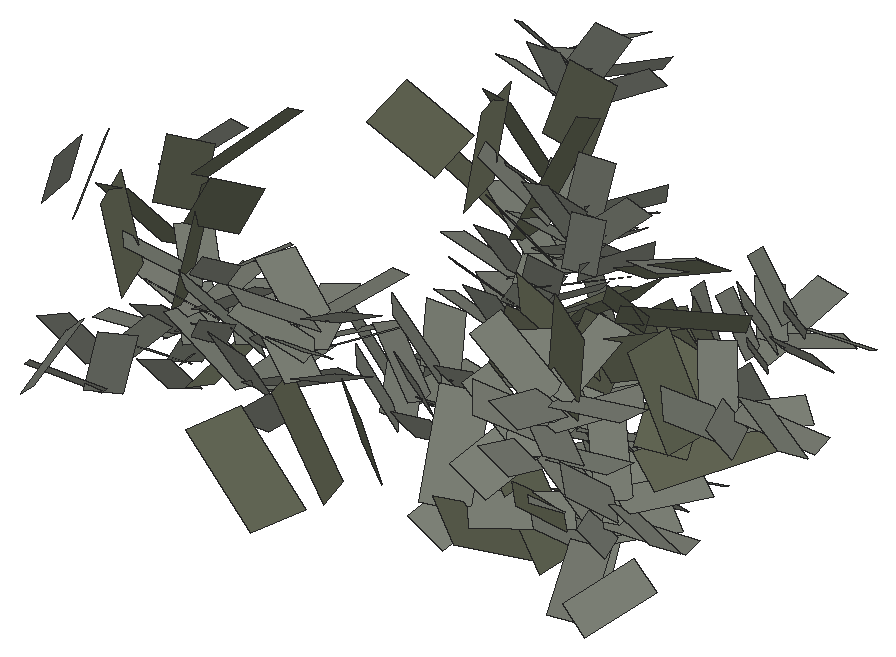
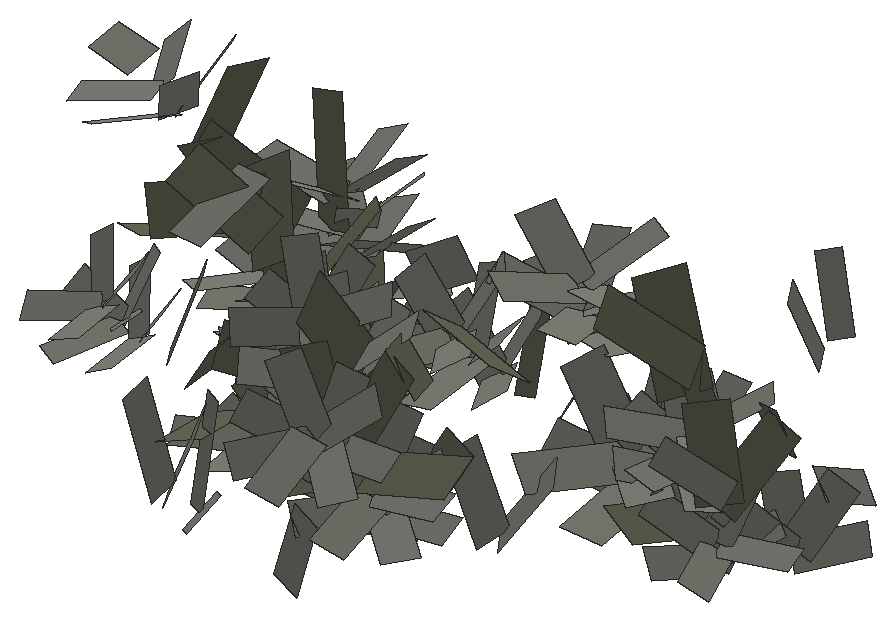
# SketchUp Ruby script. Lengths in inches.
U = 1.inch
M = Sketchup.active_model
def pt(a) = Geom::Point3d.new(a.map { |v| v * U })
def face(e, loops, mat)
  f = e.add_face(loops[0].map { |a| pt(a) })
  loops[1..].each { |l| e.add_face(l.map { |a| pt(a) }).erase! }
  f.material = f.back_material = mat if mat
  f
end
# faces: each face lists its corners as indices into pts; further lists are holes
def faces(e, pts, list, mat = nil) = list.each { |f| face(e, (f[0].is_a?(Array) ? f : [f]).map { |l| l.map { |i| pts[i] } }, mat) }
# xy, xz, yz: faces in a plane at the given z, y or x. An outline is a flat list of corners, or four numbers for a rectangle; further outlines are holes
def ring(l) = l.size == 4 ? [[l[0], l[1]], [l[2], l[1]], [l[2], l[3]], [l[0], l[3]]] : l.each_slice(2).to_a
def flat(e, list, mat, &to3) = list.each { |f| face(e, (f[0].is_a?(Array) ? f : [f]).map { |l| ring(l).map { |u, v| to3.(u, v) } }, mat) }
def xy(e, z, list, mat = nil) = flat(e, list, mat) { |x, y| [x, y, z] }
def xz(e, y, list, mat = nil) = flat(e, list, mat) { |x, z| [x, y, z] }
def yz(e, x, list, mat = nil) = flat(e, list, mat) { |y, z| [x, y, z] }
def lines(e, pts, list) = list.each { |a, b| e.add_line(pt(pts[a]), pt(pts[b])) }
# prism: a flat outline (further loops are holes) pulled along v
def prism(e, loops, v, mat = nil)
  f = face(e, loops, mat); d = Geom::Vector3d.new(v.map { |x| x * U })
  f.pushpull(f.normal.samedirection?(d) ? d.length : -d.length)
end
def box(e, o, s, mat = nil) = prism(e, [[o, [o[0] + s[0], o[1], o[2]], [o[0] + s[0], o[1] + s[1], o[2]], [o[0], o[1] + s[1], o[2]]]], [0, 0, s[2]], mat)
def at(x, y, z, deg = 0) = Geom::Transformation.translation(pt([x, y, z])) * Geom::Transformation.rotation(ORIGIN, Z_AXIS, deg.degrees)
def axes(o, x, y, z) = Geom::Transformation.new([*x, 0, *y, 0, *z, 0, *pt(o).to_a, 1])
def part(name) = M.definitions.add(name)
# library, detail: a bought-in or finely detailed component or shape, given as its bounding box
def library(name, o, s) = part(name).tap { |d| box(d.entities, o, s) }
def detail(e, o, s) = box(e.add_group.entities, o, s)
def put(e, d, t, mat = nil) = e.add_instance(d, t).tap { |i| i.material = mat if mat }
def group(e, t, mat = nil) = e.add_group.tap { |g| g.transformation = t; g.material = mat if mat }.entities
root = M.entities
M.materials.add("viburnumblaasdfas0df1w06d").color = [98, 102, 84]
M.materials.add("viburnumbladsadfasdfad0w122").color = [125, 129, 119]
c1 = part("Component\#314")
p = [[0.14,0,0],[2.58,0.05,0.25],[2.44,5.11,2.64],[0,5.05,2.39]]
faces(c1.entities,p,[[0,1,2,3]],"viburnumblaasdfas0df1w06d")
c2 = part("viburnumblad1\#2")
put(c2.entities,c1,axes([-37.25,6.23,19.31],[75.98784,0,0],[0,65.50676,0],[0,0,75.98784]))
c3 = part("Component\#315")
p = [[0.25,0,0],[2.05,0.01,0.35],[1.81,4.2,1.66],[0,4.19,1.3125]]
faces(c3.entities,p,[[0,1,2,3]],"viburnumbladsadfasdfad0w122")
c4 = part("viburnumblad2")
put(c4.entities,c3,axes([-19.23,-4.49,-32.18],[83.35428,0,0],[0,79.38502,0],[0,0,83.35428]))
put(root,c2,axes([2216.9,347.35,29.54],[-0.011,0.0051,0.00655],[-0.00551,-0.01483,0.0023],[0.00681,-0.00067,0.01196]))
put(root,c4,axes([2205.93,347.0625,36.3125],[-0.01209,-0.0034,-0.0003],[0.00332,-0.01209,0.00349],[-0.00129,0.00365,0.01095]))
put(root,c4,axes([2205.76,346.42,37.9],[-0.01088,0.00599,-0.0016],[-0.00628,-0.01045,0.00254],[-0.00013,0.00352,0.01104]))
put(root,c4,axes([2219.11,347.34,37.76],[-0.01207,0.00042,0.00346],[-0.00034,-0.01255,0.00035],[0.00347,0.00024,0.01207]))
put(root,c2,axes([2204.65,343.45,27.99],[0.00623,0.01349,0.00121],[-0.0157,0.00724,0.00014],[-0.00044,-0.00098,0.01352]))
put(root,c4,axes([2190.32,344.05,30.32],[0.00946,-0.00383,0.00571],[0.00246,0.01108,0.00318],[-0.00637,-0.00125,0.00808]))
put(root,c4,axes([2190.61,347.02,39.96],[0.00021,-0.01046,-0.0046],[0.00792,-0.00325,0.00774],[-0.00831,-0.0033,0.00712]))
put(root,c4,axes([2214.1,343.22,33.47],[0.00902,0.01086,-0.00673],[-0.00719,0.01113,0.00831],[0.01056,-0.0017,0.01141]))
put(root,c4,axes([2218.1,347.48,34.8125],[-0.0126,0.00044,0.00361],[-0.00031,-0.0113,0.00032],[0.00347,0.00024,0.01207]))
put(root,c4,axes([2205.46,347.33,34.83],[-0.00597,-0.01037,0.00113],[0.01154,-0.00613,0.0032],[-0.00222,0.00293,0.01099]))
put(root,c2,axes([2207.0625,345,29.67],[-0.00512,0.01258,-0.00225],[-0.01225,-0.00318,0.00944],[0.00707,0.00483,0.00942]))
put(root,c2,axes([2217.31,348.43,31.83],[-0.01089,-0.0066,0.00527],[0.00777,-0.0139,-0.00135],[0.00514,0.00164,0.01268]))
put(root,c4,axes([2221.26,344.42,30.01],[0.00733,0.00034,-0.00907],[0.00348,0.00978,0.00299],[0.00808,-0.00497,0.00546]))
put(root,c4,axes([2220.3,344.48,29.09],[0.00746,0.0085,-0.0048],[-0.00195,0.00645,0.00799],[0.00881,-0.00455,0.00477]))
put(root,c4,axes([2214.24,344.98,33.36],[0.00842,-0.01125,-0.00685],[0.01063,0.01127,-0.00543],[0.00843,-0.00165,0.01307]))
put(root,c2,axes([2208.35,346.97,30.46],[-0.01166,0.00571,0.00452],[-0.00151,-0.01177,0.01017],[0.0071,0.00732,0.00793]))
put(root,c4,axes([2205.3,345.74,36.45],[-0.0033,0.01188,-0.00196],[-0.01112,-0.00285,0.00099],[0.00058,0.00262,0.01122]))
put(root,c4,axes([2218.33,346.89,36.22],[-0.008,0.00913,0.00324],[-0.00789,-0.00792,0.00285],[0.00448,-0.00024,0.01173]))
put(root,c4,axes([2218.32,348.36,36.4],[-0.00907,-0.00853,0.00165],[0.00877,-0.00968,-0.00184],[0.0024,-0.00017,0.01233]))
put(root,c4,axes([2205.61,347.97,37.66],[-0.00622,-0.0108,0.00117],[0.01069,-0.00568,0.00296],[-0.00222,0.00293,0.01099]))
put(root,c4,axes([2228.56,348.54,39.8],[-0.00908,-0.00254,0.00688],[0.00302,-0.01141,-0.00024],[0.00679,0.00165,0.00837]))
put(root,c4,axes([2221.14,348.53,31.72],[-0.00974,-0.00261,0.006],[0.00353,-0.01123,0.00072],[0.00551,0.00254,0.00899]))
put(root,c4,axes([2220.21,347.85,30.78],[-0.00853,0.00601,0.00433],[-0.00446,-0.01051,0.00545],[0.00645,0.00235,0.00846]))
put(root,c4,axes([2212.86,344.05,32],[0.01184,-0.00027,-0.00922],[0.00172,0.01671,0.00172],[0.00948,-0.00223,0.01224]))
put(root,c4,axes([2227.48,347.97,38.95],[-0.00764,0.00611,0.00552],[-0.0043,-0.01063,0.00535],[0.00765,0.00146,0.00773]))
put(root,c4,axes([2221.76,347.79,33.03],[-0.00889,0.00626,0.00451],[-0.00413,-0.00973,0.00504],[0.00645,0.00235,0.00846]))
put(root,c4,axes([2215.02,344.33,35.29],[0.01234,-0.00028,-0.00961],[0.00159,0.01547,0.00159],[0.00948,-0.00223,0.01224]))
put(root,c4,axes([2217.81,346.48,38.03],[0.00076,0.01249,0.00112],[-0.01157,0.00026,0.0049],[0.00485,-0.00133,0.01151]))
put(root,c4,axes([2204.4,345.6,35.14],[0.00564,0.00974,-0.00221],[-0.01091,0.00622,-0.00021],[0.00111,0.00263,0.01119]))
put(root,c4,axes([2192.31,347.93,29.6],[-0.00614,0.00518,-0.0082],[-0.00794,-0.00715,0.00088],[-0.00475,0.00709,0.00648]))
put(root,c4,axes([2190.82,347.36,38.47],[0.00662,-0.00815,0.00069],[0.00514,0.00494,0.00894],[-0.00725,-0.00529,0.00709]))
put(root,c4,axes([2217.05,346.68,35.125],[0.00022,0.01156,-0.00012],[-0.01157,0.00026,0.0049],[0.0049,0.00003,0.01157]))
put(root,c4,axes([2229.24,349.17,41],[-0.00489,-0.00995,0.00397],[0.00876,-0.00628,-0.0047],[0.00608,0.00102,0.00892]))
put(root,c2,axes([2217.91,347.02,29.08],[0.00107,0.01287,0.00071],[-0.01171,0.00034,0.00907],[0.0079,-0.00141,0.00892]))
put(root,c4,axes([2221.62,349.27,32.95],[-0.00489,-0.00995,0.00397],[0.00954,-0.00607,-0.00338],[0.00477,0.0019,0.00949]))
put(root,c4,axes([2218.31,348.66,38.125],[-0.00076,-0.01249,-0.00112],[0.01239,-0.00058,-0.00197],[0.0019,-0.00123,0.01236]))
put(root,c4,axes([2204.76,347.85,36.15],[0.0033,-0.01188,0.00196],[0.01189,0.00365,0.00167],[-0.00236,0.00179,0.01115]))
put(root,c4,axes([2217.17,348.73,35.17],[-0.00073,-0.01199,-0.00108],[0.01339,-0.00063,-0.00213],[0.0019,-0.00123,0.01236]))
put(root,c4,axes([2220.49,347.47,32.1875],[-0.00283,0.01146,0.00038],[-0.0094,-0.00257,0.00741],[0.00704,0.00146,0.00821]))
put(root,c2,axes([2224.92,347.37,37.5],[0.00184,0.01273,0.00122],[-0.0105,0.00029,0.01027],[0.00896,-0.0024,0.00784]))
put(root,c4,axes([2191.86,349.27,30.3],[-0.01,-0.00241,-0.00568],[-0.00201,-0.00892,0.00667],[-0.00557,0.00722,0.00577]))
put(root,c4,axes([2192.36,349.06,28.86],[-0.008,-0.00859,0.00017],[0.00566,-0.00462,0.00938],[-0.00647,0.00667,0.0055]))
put(root,c4,axes([2204.18,346.25,37.82],[0.00622,0.0108,-0.00117],[-0.01091,0.00622,-0.00021],[0.00044,0.00147,0.01138]))
put(root,c4,axes([2208.94,349.56,32.23],[-0.00734,-0.00647,0.00686],[0.01022,-0.00834,0.00267],[0.00284,0.00722,0.00872]))
put(root,c2,axes([2218.16,348.42,36.08],[-0.01355,0.00411,0.00465],[0.00135,-0.01078,0.01345],[0.00609,0.01091,0.00813]))
put(root,c4,axes([2208.95,348.22,33.07],[-0.00945,0.00892,-0.00145],[-0.0064,-0.00533,0.00736],[0.00487,0.007,0.00802]))
put(root,c4,axes([2200.49,349.96,31.1],[-0.01458,-0.00076,0.00047],[0.00121,-0.01217,0.00796],[0.00032,0.00837,0.01162]))
put(root,c4,axes([2209.86,349.68,33.51],[-0.01181,0.00128,0.00407],[0.00154,-0.01046,0.00743],[0.00382,0.0075,0.00815]))
put(root,c4,axes([2199.99,350.08,29.27],[-0.0086,-0.00967,0.00326],[0.01109,-0.00774,0.00569],[-0.00192,0.00675,0.01234]))
put(root,c4,axes([2219.47,346.63,29.39],[0.00909,0.00791,-0.00471],[-0.00403,0.00937,0.00796],[0.00828,-0.00412,0.00905]))
put(root,c4,axes([2196.97,350.23,33.79],[-0.01133,0.00035,-0.0015],[-0.0009,-0.01068,0.0043],[-0.00126,0.00434,0.0105]))
put(root,c4,axes([2203.76,346.59,36.26],[0.01209,0.0034,0.0003],[-0.00342,0.01218,-0.00058],[-0.00049,0.00075,0.01143]))
put(root,c4,axes([2216.64,346.95,36.74],[0.00907,0.00853,-0.00165],[-0.0076,0.009,0.00473],[0.00435,-0.00239,0.01154]))
put(root,c4,axes([2196.89,350.67,32.32],[-0.00757,-0.0073,-0.00011],[0.00727,-0.00761,0.00446],[-0.00317,0.00314,0.01053]))
put(root,c4,axes([2216.97,348.53,36.82],[0.008,-0.00913,-0.00324],[0.00942,0.00831,-0.00017],[0.00227,-0.00232,0.01214]))
put(root,c4,axes([2227.64,349.54,40.45],[0.00217,-0.01153,-0.00126],[0.00998,0.00257,-0.00587],[0.00594,-0.00007,0.00905]))
put(root,c4,axes([2204.03,347.81,37.58],[0.01088,-0.00599,0.0016],[0.00606,0.01099,0.00021],[-0.00165,0.00089,0.01133]))
put(root,c4,axes([2220.1,349.52,32.21],[0.00283,-0.01146,-0.00038],[0.01049,0.00275,-0.00491],[0.00467,0.00082,0.00968]))
put(root,c4,axes([2218.96,347.65,31.57],[0.0051,0.01038,-0.00415],[-0.00729,0.00572,0.00502],[0.00694,0.00038,0.0084]))
put(root,c4,axes([2226.33,347.78,39.87],[0.0051,0.01038,-0.00415],[-0.00633,0.00571,0.00604],[0.00802,-0.00053,0.00751]))
put(root,c4,axes([2199.9,349.96,33.125],[-0.01112,0.00864,-0.0042],[-0.00937,-0.00881,0.00635],[0.00161,0.00797,0.01181]))
put(root,c4,axes([2220.49,347.71,33.79],[0.00489,0.00995,-0.00397],[-0.0081,0.00635,0.00558],[0.00694,0.00038,0.0084]))
put(root,c4,axes([2196.19,349.92,35.3],[-0.00749,0.00804,-0.00315],[-0.00863,-0.00712,0.00235],[-0.00031,0.00392,0.01074]))
put(root,c4,axes([2210.16,349.75,35.19],[-0.00905,0.00854,-0.00139],[-0.00711,-0.00593,0.00818],[0.00487,0.007,0.00802]))
put(root,c4,axes([2210.29,351.07,34.36],[-0.00765,-0.00673,0.00714],[0.00947,-0.00772,0.00247],[0.00284,0.00722,0.00872]))
put(root,c4,axes([2217.01,347.8,38.4],[0.01207,-0.00042,-0.00346],[0.00117,0.01224,0.00258],[0.00328,-0.0028,0.0118]))
put(root,c4,axes([2196.53,351.29,34.96],[-0.00853,-0.00755,0.00102],[0.00727,-0.00761,0.00446],[-0.00226,0.00398,0.01048]))
put(root,c2,axes([2193.4,348.24,34.14],[0.00699,0.00088,0.01038],[-0.00621,0.01278,0.0031],[-0.00893,-0.00592,0.00652]))
put(root,c4,axes([2195.03,351.27,29.09],[-0.00996,-0.0034,-0.00378],[0.00101,-0.00837,0.00457],[-0.00471,0.00422,0.00764]))
put(root,c2,axes([2222.75,347.77,36.74],[0.00961,0.00746,-0.00443],[-0.00604,0.01187,0.00656],[0.0068,-0.00274,0.00947]))
put(root,c4,axes([2200.07,351.59,32.32],[-0.0095,-0.00972,0.00486],[0.01109,-0.00774,0.00569],[-0.0009,0.00784,0.01189]))
put(root,c4,axes([2219.39,348.11,32.74],[0.00974,0.00261,-0.006],[-0.00192,0.01057,0.00135],[0.0062,-0.00026,0.0089]))
put(root,c4,axes([2199.07,348.9,31.64],[-0.00115,0.01298,-0.0064],[-0.01441,0.00008,0.00199],[0.00223,0.00688,0.01234]))
put(root,c4,axes([2209.04,348.81,34.35],[-0.00099,0.0108,-0.00603],[-0.01031,0.00186,0.00471],[0.00538,0.00602,0.00839]))
put(root,c4,axes([2218.83,348.92,31.61],[0.00761,-0.00572,-0.00506],[0.00557,0.01001,-0.00285],[0.00619,-0.00075,0.00889]))
put(root,c4,axes([2208.92,350.72,33.31],[0.00099,-0.0108,0.00603],[0.0122,-0.00051,-0.00294],[0.0025,0.00634,0.00938]))
put(root,c4,axes([2191.27,350.1,29.27],[-0.00132,-0.00974,0.00592],[0.00922,0.00313,0.00644],[-0.00695,0.00574,0.0058]))
put(root,c4,axes([2226.27,349.04,39.97],[0.00664,-0.00572,-0.00612],[0.00571,0.0099,-0.00294],[0.00728,-0.00165,0.00803]))
put(root,c2,axes([2196.22,351.8,36.53],[-0.00965,-0.00928,0.0022],[0.01068,-0.00958,0.00645],[-0.00246,0.00545,0.01217]))
put(root,c4,axes([2195.75,349.43,33.86],[0.00073,0.01102,-0.00295],[-0.01141,0.00071,-0.00016],[0.00003,0.00295,0.01104]))
put(root,c4,axes([2220.34,349.19,33.7],[0.00889,-0.00626,-0.00451],[0.00557,0.01001,-0.00285],[0.00526,-0.00007,0.00943]))
put(root,c4,axes([2194.45,351.25,30.15],[-0.00794,0.00459,-0.00546],[-0.00557,-0.00804,0.00123],[-0.00382,0.00415,0.0081]))
put(root,c2,axes([2195.05,350.27,33.1875],[0.00608,-0.01136,0.00423],[0.00607,0.0078,0.01224],[-0.01094,-0.0031,0.0074]))
put(root,c4,axes([2207.7,348.55,33.5],[0.00649,0.00565,-0.00743],[-0.0085,0.00924,-0.00029],[0.00584,0.00584,0.00823]))
put(root,c4,axes([2194.01,352.22,31.1],[-0.00954,-0.00326,-0.00362],[0.00113,-0.0093,0.00507],[-0.00471,0.00422,0.00764]))
put(root,c4,axes([2195.92,351.36,33.32],[-0.00073,-0.01102,0.00295],[0.01017,0.00002,0.00259],[-0.00273,0.00304,0.01068]))
put(root,c4,axes([2198.92,351.16,30.47],[0.00115,-0.01298,0.0064],[0.01333,0.00146,0.00097],[-0.00132,0.00669,0.01246]))
put(root,c4,axes([2194.16,352.37,29.65],[-0.00555,-0.00919,0.00035],[0.0077,-0.00439,0.00674],[-0.00547,0.00359,0.00747]))
put(root,c2,axes([2221.17,349.22,35.06],[0.01127,-0.00662,-0.00498],[0.00702,0.01432,-0.0031],[0.00548,-0.00011,0.01154]))
put(root,c2,axes([2217.87,351.27,37.12],[-0.00474,-0.00612,0.0114],[0.01476,-0.00511,0.0034],[0.00234,0.01154,0.00716]))
put(root,c4,axes([2195.49,349.42,32.36],[0.00819,0.00724,-0.00098],[-0.00821,0.00902,-0.00193],[-0.00044,0.00202,0.01125]))
put(root,c4,axes([2193.15,351.17,31.03],[-0.00169,0.00975,-0.0041],[-0.01002,-0.00286,-0.00259],[-0.00334,0.00343,0.00858]))
put(root,c4,axes([2195.7,350.83,32.04],[0.00782,-0.00839,0.00329],[0.00747,0.00707,0.00029],[-0.00239,0.00208,0.01099]))
put(root,c4,axes([2207.78,350.03,34.18],[0.01181,-0.00128,-0.00407],[-0.00051,0.0116,-0.00495],[0.00406,0.00486,0.00962]))
put(root,c4,axes([2214.95,352.62,31.57],[-0.00706,0.00732,-0.0001],[-0.00736,-0.00703,0.00431],[0.00303,0.00306,0.01018]))
put(root,c4,axes([2215.61,353.55,32.53],[-0.01066,0.00071,0.00285],[0.00002,-0.00983,0.00251],[0.00294,0.00264,0.01033]))
put(root,c4,axes([2194.8,350.2,35.05],[0.00853,0.00755,-0.00102],[-0.0076,0.00835,-0.00179],[-0.00044,0.00202,0.01125]))
put(root,c4,axes([2215.1,353.77,31.29],[-0.00812,-0.00757,0.00318],[0.00684,-0.00722,0.00028],[0.00201,0.00231,0.01062]))
put(root,c2,axes([2195.59,349.71,29.32],[0.01125,-0.00276,0.00479],[0.00395,0.01395,-0.00123],[-0.00436,0.00225,0.01154]))
put(root,c4,axes([2208.67,350.14,35.57],[0.00765,0.00673,-0.00714],[-0.0085,0.00924,-0.00029],[0.00504,0.00514,0.00906]))
put(root,c4,axes([2208.8,351.46,34.73],[0.00905,-0.00854,0.00139],[0.00807,0.00744,-0.006],[0.00301,0.00536,0.00976]))
put(root,c2,axes([2216.04,353.26,35.63],[-0.00897,0.00933,0.00213],[-0.00926,-0.01033,0.00624],[0.00527,0.00238,0.01177]))
put(root,c4,axes([2194.99,350.4,33.48],[0.01133,-0.00035,0.0015],[0.00059,0.01187,-0.00167],[-0.00144,0.00165,0.01122]))
put(root,c4,axes([2195.13,351.57,34.71],[0.00749,-0.00804,0.00315],[0.0083,0.00786,0.00032],[-0.00239,0.00208,0.01099]))
put(root,c4,axes([2215.54,352.96,34.12],[-0.0073,0.00825,0.00099],[-0.00736,-0.00703,0.00431],[0.00384,0.00219,0.01013]))
put(root,c2,axes([2192.51,353.63,33.79],[-0.01098,0.00138,-0.00403],[-0.00375,-0.01153,0.00597],[-0.00261,0.00614,0.00861]))
put(root,c4,axes([2198.0625,350.14,33.05],[0.0095,0.00972,-0.00486],[-0.01098,0.00941,-0.00264],[0.00181,0.00573,0.01291]))
put(root,c4,axes([2197.91,349.95,31.09],[0.01458,0.00076,-0.00047],[-0.00114,0.0144,-0.00508],[0.00059,0.00521,0.01318]))
put(root,c4,axes([2215.82,354.3125,33.88],[-0.00778,-0.00725,0.00304],[0.0076,-0.00802,0.00031],[0.00201,0.00231,0.01062]))
put(root,c4,axes([2193.14,352.99,30.41],[0.00169,-0.00975,0.0041],[0.00892,0.0036,0.00459],[-0.00566,0.00263,0.0077]))
put(root,c2,axes([2214.02,353.87,28.66],[-0.00267,-0.01088,0.00464],[0.01349,-0.00382,-0.00119],[0.00218,0.00422,0.01116]))
put(root,c4,axes([2198.23,351.77,32.24],[0.01112,-0.00864,0.0042],[0.00948,0.01048,-0.0033],[-0.0007,0.0056,0.01299]))
put(root,c2,axes([2194.29,352.42,38.4375],[0.00364,-0.01074,0.00535],[0.01254,0.00622,0.00396],[-0.00521,0.00362,0.01082]))
put(root,c2,axes([2216.64,355.125,37.48],[-0.01039,-0.00352,0.00517],[0.00601,-0.01213,0.00383],[0.0035,0.00504,0.01046]))
put(root,c4,axes([2193.0625,352.1,29.22],[0.00794,-0.00459,0.00546],[0.00496,0.0095,0.00066],[-0.00518,0.00191,0.00818]))
put(root,c4,axes([2214.52,352.53,32.99],[0.00034,0.01095,-0.00145],[-0.01033,0.00087,0.00416],[0.0042,0.00122,0.01016]))
put(root,c4,axes([2214.69,354.45,32.68],[-0.00034,-0.01095,0.00145],[0.01148,-0.00057,-0.00162],[0.0016,0.00139,0.01085]))
put(root,c4,axes([2192.28,351.94,30.34],[0.00954,0.00326,0.00362],[-0.00223,0.01005,-0.00307],[-0.00429,0.00184,0.00864]))
put(root,c2,axes([2214.56,354.39,32.4],[-0.01099,-0.00588,0.00409],[0.00754,-0.00587,0.01184],[-0.00299,0.01058,0.00715]))
put(root,c2,axes([2217.08,352.8,39.02],[0.00672,-0.00769,0.00925],[0.01396,0.00492,-0.00605],[0.00006,0.01062,0.00878]))
put(root,c2,axes([2191.375,355.29,34.48],[-0.00937,-0.00701,0.00111],[0.00657,-0.00694,0.00934],[-0.00422,0.00731,0.00713]))
put(root,c4,axes([2216.59,355.25,28.98],[-0.00889,0.00537,0.00033],[-0.00425,-0.00744,0.00652],[0.00347,0.00529,0.00723]))
put(root,c4,axes([2213.74,353.97,31.6],[0.00701,-0.00792,-0.00095],[0.00872,0.00794,-0.00187],[0.00195,0.00042,0.01087]))
put(root,c4,axes([2217.19,356.24,29.72],[-0.00943,-0.00164,0.00397],[0.00349,-0.00863,0.00444],[0.00255,0.00548,0.00745]))
put(root,c4,axes([2214.23,353.29,34.45],[0.00778,0.00725,-0.00304],[-0.00689,0.00834,0.00227],[0.00379,0.0003,0.01038]))
put(root,c4,axes([2203.53,356.57,28.99],[-0.01014,-0.00518,0.00703],[0.00849,-0.00835,0.00609],[0.00203,0.00907,0.00962]))
put(root,c4,axes([2216.34,356.32,28.5625],[-0.00444,-0.00768,0.00528],[0.00919,-0.00479,0.00064],[0.00185,0.00501,0.00791]))
put(root,c4,axes([2214.5,354.64,34.2],[0.0073,-0.00825,-0.00099],[0.00807,0.00735,-0.00173],[0.00195,0.00042,0.01087]))
put(root,c4,axes([2213.75,353.72,33.06],[0.01066,-0.00071,-0.00285],[0.00069,0.01103,-0.00015],[0.00286,-0.00003,0.01068]))
put(root,c4,axes([2203.08,355.35,30.07],[-0.00818,0.0094,-0.00487],[-0.00969,-0.00417,0.00823],[0.00426,0.00856,0.00935]))
put(root,c2,axes([2216,356.23,39.34],[-0.00272,-0.01048,0.00546],[0.01366,-0.00332,0.00044],[0.00096,0.00539,0.01082]))
put(root,c4,axes([2216.45,355.4,30.39],[-0.00315,0.00923,-0.0035],[-0.009,-0.00109,0.00491],[0.00408,0.00455,0.00739]))
put(root,c4,axes([2217.16,354.28,42.04],[0.01174,-0.00224,-0.0016],[0.00091,0.0107,-0.00829],[0.00274,0.00736,0.0098]))
put(root,c2,axes([2207.91,357.15,28.37],[-0.01202,0.00402,-0.00269],[-0.00561,-0.01134,0.00795],[0.00019,0.00723,0.00942]))
put(root,c4,axes([2215.51,354.97,29.47],[0.00444,0.00768,-0.00528],[-0.00777,0.00538,0.00119],[0.00402,0.0037,0.00783]))
put(root,c4,axes([2189.34,356.55,35.8],[0.00099,-0.00884,0.00502],[0.00961,0.00407,0.00487],[-0.00586,0.00398,0.00703]))
put(root,c4,axes([2216.18,357.07,29.65],[0.00315,-0.00923,0.0035],[0.00972,0.00216,-0.00297],[0.00178,0.00415,0.00836]))
put(root,c4,axes([2211.74,358.49,37.51],[-0.00788,-0.0064,0.00067],[0.00477,-0.00497,0.00864],[-0.00511,0.00701,0.00686]))
put(root,c2,axes([2212.6,355.98,33.32],[0.00085,-0.00676,0.01003],[0.01236,0.00601,0.00299],[-0.00572,0.00864,0.0063]))
put(root,c4,axes([2211.42,358.69,38.95],[-0.01012,-0.0002,-0.00445],[-0.00314,-0.00766,0.00749],[-0.00319,0.00804,0.00689]))
put(root,c4,axes([2208.82,359.54,35.09],[-0.00994,-0.00547,0.00222],[0.00636,-0.00933,0.00551],[-0.00082,0.00596,0.01103]))
put(root,c2,axes([2219.41,357.95,33.65],[-0.00677,0.00906,0.00107],[-0.00671,-0.00636,0.00903],[0.00707,0.00408,0.0069]))
put(root,c4,axes([2215.4375,356.23,30.3125],[0.00943,0.00164,-0.00397],[-0.00277,0.00969,-0.0025],[0.00332,0.00323,0.0083]))
put(root,c4,axes([2209.03,359.3,36.75],[-0.01209,0.00339,-0.00041],[-0.00309,-0.0102,0.00689],[0.00151,0.00666,0.01054]))
put(root,c2,axes([2207.21,359.1875,29.2],[-0.01137,-0.00525,0.00325],[0.00699,-0.00886,0.00961],[-0.00151,0.00884,0.00798]))
put(root,c2,axes([2217.8125,356.84,32.98],[0.00134,0.01062,-0.0039],[-0.01115,0.00362,0.00577],[0.00594,0.00252,0.00833]))
put(root,c4,axes([2220.63,359.91,34.93],[-0.00855,-0.00095,0.00486],[0.00394,-0.00929,0.00471],[0.00385,0.00566,0.0068]))
put(root,c4,axes([2210.29,359.03,40.13],[-0.00525,0.00588,-0.00776],[-0.00943,-0.00525,0.0024],[-0.00241,0.00775,0.0075]))
put(root,c2,axes([2204.18,357.16,40.14],[0.00447,0.01094,0.00709],[-0.01215,0.00867,-0.00572],[-0.00776,-0.00379,0.01074]))
put(root,c4,axes([2210.17,358.02,38.99],[0.0027,0.00851,-0.00652],[-0.01047,0.00066,-0.00347],[-0.00228,0.00703,0.00822]))
put(root,c4,axes([2206.51,360.17,31.7],[-0.01201,-0.00131,-0.00224],[-0.00042,-0.0083,0.00649],[-0.00262,0.00705,0.00788]))
put(root,c2,axes([2207.51,358.23,29.77],[0.00221,-0.01095,0.00807],[0.01572,0.00285,-0.00044],[-0.00114,0.008,0.01116]))
put(root,c4,axes([2209.03,360.73,37.84],[-0.01083,-0.00527,0.00359],[0.00636,-0.00933,0.00551],[0.00035,0.00657,0.01071]))
put(root,c4,axes([2210.85,360.09,39.42],[-0.00906,-0.00616,0.00146],[0.00477,-0.00497,0.00864],[-0.00416,0.00772,0.00674]))
put(root,c4,axes([2210.29,357.42,37.65],[0.0087,0.00591,-0.0014],[-0.00609,0.00723,-0.0073],[-0.00288,0.00629,0.00863]))
put(root,c2,axes([2211.15,356.45,34.99],[0.00897,-0.0006,0.00814],[0.00562,0.01175,-0.00532],[-0.00657,0.00665,0.00773]))
put(root,c4,axes([2221.21,359.88,36.11],[-0.00853,0.00582,0.00111],[-0.0037,-0.00695,0.00724],[0.00473,0.00542,0.00649]))
put(root,c4,axes([2210.6875,359.5,37.83],[-0.0027,-0.00851,0.00652],[0.00882,0.00097,0.00492],[-0.00475,0.00698,0.00714]))
put(root,c4,axes([2210.73,358.52,36.89],[0.00548,-0.00614,0.0081],[0.00771,0.00628,-0.00046],[-0.00462,0.00625,0.00786]))
put(root,c4,axes([2208.37,359.45,38.52],[-0.00627,0.01006,-0.00416],[-0.01061,-0.00457,0.00494],[0.00244,0.00598,0.01078]))
put(root,c4,axes([2221.96,360.87,36.73],[-0.00891,-0.00099,0.00506],[0.00365,-0.0086,0.00436],[0.00385,0.00566,0.0068]))
put(root,c2,axes([2215.93,356.77,31.5],[0.01113,0.00289,-0.00438],[-0.00454,0.01328,-0.00273],[0.00348,0.00335,0.01016]))
put(root,c4,axes([2208.15,360.7,36.125],[-0.00322,-0.01084,0.00548],[0.01114,-0.00248,0.00163],[-0.00036,0.00575,0.01116]))
put(root,c4,axes([2220.95,360.94,35.68],[-0.00407,-0.00723,0.00605],[0.00898,-0.00522,-0.00021],[0.0032,0.00525,0.00736]))
put(root,c4,axes([2220.04,359.07,35.74],[-0.00329,0.00963,-0.00365],[-0.00749,-0.00039,0.00532],[0.00532,0.00466,0.00661]))
put(root,c4,axes([2206.06,360.49,32.91],[-0.00804,0.00619,-0.0059],[-0.0078,-0.0066,0.00358],[-0.00163,0.0068,0.00829]))
put(root,c4,axes([2205.5,359.44,32],[0.00025,0.00856,-0.00655],[-0.01174,-0.00053,-0.00107],[-0.00121,0.00703,0.00818]))
put(root,c4,axes([2207.56,360,34.88],[0.00655,-0.0105,0.00435],[0.00979,0.0053,-0.00197],[-0.0002,0.0047,0.01165]))
put(root,c4,axes([2207.54,358.83,37.125],[0.00322,0.01084,-0.00548],[-0.01186,0.00402,0.00097],[0.00259,0.00493,0.01126]))
put(root,c4,axes([2205.97,361.66,32.18],[-0.00824,-0.00797,0.00286],[0.00803,-0.0057,0.00726],[-0.00361,0.00659,0.00792]))
put(root,c4,axes([2206.01,361.79,33.79],[-0.01151,-0.00126,-0.00215],[-0.00046,-0.00922,0.00721],[-0.00262,0.00705,0.00788]))
put(root,c4,axes([2209.67,358.73,38.08],[0.01012,0.0002,0.00445],[0.00236,0.00977,-0.0058],[-0.00385,0.00596,0.00848]))
put(root,c2,axes([2206.92,359.79,36.31],[0.00407,-0.01295,0.00616],[0.01043,0.00846,0.01089],[-0.01117,0.00115,0.0098]))
put(root,c2,axes([2204.8,358.3,37.92],[0.00927,0.00064,0.01018],[-0.00266,0.0157,0.00144],[-0.00994,-0.00253,0.00921]))
put(root,c4,axes([2221.27,360.1,37.51],[-0.00315,0.00923,-0.0035],[-0.00832,-0.00043,0.00591],[0.00532,0.00466,0.00661]))
put(root,c4,axes([2216.14,361.33,29.02],[-0.01262,0.00712,0.00249],[-0.00199,-0.00788,0.01243],[0.00728,0.01023,0.00765]))
put(root,c4,axes([2209.09,359.1875,39.44],[0.00906,0.00616,-0.00146],[-0.00564,0.00669,-0.00676],[-0.00288,0.00629,0.00863]))
put(root,c4,axes([2205.58,361.02,30.9],[-0.00014,-0.00961,0.00594],[0.01198,0.00212,0.00345],[-0.00404,0.00568,0.00838]))
put(root,c4,axes([2207.02,358.64,35.54],[0.01039,0.00506,-0.00344],[-0.00658,0.01149,-0.00298],[0.00188,0.00411,0.01172]))
put(root,c2,axes([2206.72,358.4,32.2],[0.0119,-0.00534,0.00444],[0.00766,0.01326,-0.00459],[-0.00215,0.00555,0.01243]))
put(root,c4,axes([2209.64,360.25,38.72],[0.00525,-0.00588,0.00776],[0.00856,0.00697,-0.00051],[-0.00462,0.00625,0.00786]))
put(root,c4,axes([2220.1875,359.67,36.73],[0.00407,0.00723,-0.00605],[-0.00729,0.00582,0.00182],[0.00528,0.00383,0.00709]))
put(root,c4,axes([2220.98,361.75,36.74],[0.00315,-0.00923,0.0035],[0.00936,0.00154,-0.00413],[0.00315,0.00442,0.00785]))
put(root,c4,axes([2219.21,359.83,35.83],[0.00769,0.00057,-0.00539],[-0.00261,0.00972,-0.00258],[0.00555,0.0035,0.00706]))
put(root,c4,axes([2204.81,360.93,34.02],[0.00014,0.01001,-0.00619],[-0.01174,-0.00053,-0.00107],[-0.00123,0.00599,0.0089]))
put(root,c4,axes([2207.6,361.38,37.67],[0.00627,-0.01006,0.00416],[0.01088,0.00589,-0.00218],[-0.0002,0.0047,0.01165]))
put(root,c4,axes([2206.9375,360,36.6],[0.01209,-0.00339,0.00041],[0.0035,0.01198,-0.00427],[0.00073,0.00402,0.01188]))
put(root,c4,axes([2216.85,363.24,29.57],[-0.01093,-0.00132,0.00974],[0.00771,-0.01018,0.00728],[0.00609,0.01052,0.00826]))
put(root,c4,axes([2219.76,360.99,36.25],[0.00853,-0.00582,-0.00111],[0.00461,0.00781,-0.00517],[0.00374,0.00366,0.00797]))
put(root,c4,axes([2204.43,360.33,32.64],[0.00824,0.00797,-0.00286],[-0.00838,0.00693,-0.00484],[-0.00165,0.00508,0.00936]))
put(root,c4,axes([2206.9375,360.11,38.35],[0.01083,0.00527,-0.00359],[-0.00609,0.01064,-0.00276],[0.00188,0.00411,0.01172]))
put(root,c4,axes([2205.18,362.73,32.99],[-0.00014,-0.01001,0.00619],[0.0111,0.00196,0.00319],[-0.00404,0.00568,0.00838]))
put(root,c4,axes([2220.29,360.98,37.51],[0.00891,0.00099,-0.00506],[-0.00261,0.00972,-0.00258],[0.00462,0.00341,0.00766]))
put(root,c4,axes([2204.67,361.625,31.89],[0.00804,-0.00619,0.0059],[0.00785,0.00862,-0.00178],[-0.00364,0.00486,0.00899]))
put(root,c2,axes([2204.56,361.83,35.3],[-0.00083,0.01216,-0.00686],[-0.01618,-0.00142,-0.00053],[-0.00101,0.00652,0.01095]))
put(root,c4,axes([2216.23,362.27,31.02],[-0.00691,0.01139,-0.00621],[-0.01,-0.00019,0.01077],[0.00826,0.00929,0.00783]))
put(root,c4,axes([2214.63,361.38,30.14],[0.00284,0.00899,-0.01128],[-0.01167,0.00819,0.00358],[0.00847,0.00827,0.00872]))
put(root,c2,axes([2205.23,364.15,36.56],[-0.01186,0.00394,-0.00337],[-0.00604,-0.00999,0.00917],[0.00026,0.00862,0.00831]))
put(root,c4,axes([2203.98,361.87,33.22],[0.01151,0.00126,0.00215],[-0.00018,0.01065,-0.00509],[-0.00265,0.00461,0.00939]))
put(root,c4,axes([2208.26,365.01,29.55],[-0.01122,0.00147,-0.00326],[-0.00368,-0.004,0.01025],[0.00008,0.01052,0.00323]))
put(root,c2,axes([2204.58,366.32,37.09],[-0.01156,-0.00444,0.00366],[0.00659,-0.0076,0.0107],[-0.00137,0.01006,0.00666]))
put(root,c4,axes([2203.87,367.7,39.41],[-0.01201,-0.00131,-0.00224],[-0.00075,-0.00731,0.00743],[-0.00252,0.0083,0.00677]))
put(root,c4,axes([2202.84,367.04,39.77],[0.00059,0.00756,-0.00753],[-0.01174,-0.00037,-0.00119],[-0.00112,0.00828,0.00709]))
put(root,c4,axes([2203.42,368.21,40.55],[-0.00777,0.00552,-0.00673],[-0.00804,-0.00584,0.00423],[-0.00155,0.00808,0.00722]))
put(root,c4,axes([2203.37,369.27,39.67],[-0.0085,-0.0073,0.00369],[0.00776,-0.00483,0.008],[-0.00353,0.00786,0.00685]))
put(root,c4,axes([2202.99,368.45,38.49],[-0.0005,-0.0087,0.00708],[0.01199,0.0023,0.00332],[-0.00399,0.00704,0.00741]))
put(root,c4,axes([2201.79,368.05,40.26],[0.0085,0.0073,-0.00369],[-0.00811,0.00643,-0.0058],[-0.00164,0.00652,0.00849]))
put(root,c4,axes([2202.08,369.23,39.375],[0.00777,-0.00552,0.00673],[0.00812,0.00813,-0.00272],[-0.00362,0.0063,0.00812]))
put(root,c4,axes([2201.38,369.69,40.63],[0.01151,0.00126,0.00215],[0.0002,0.00988,-0.00637],[-0.00265,0.00609,0.00857]))
